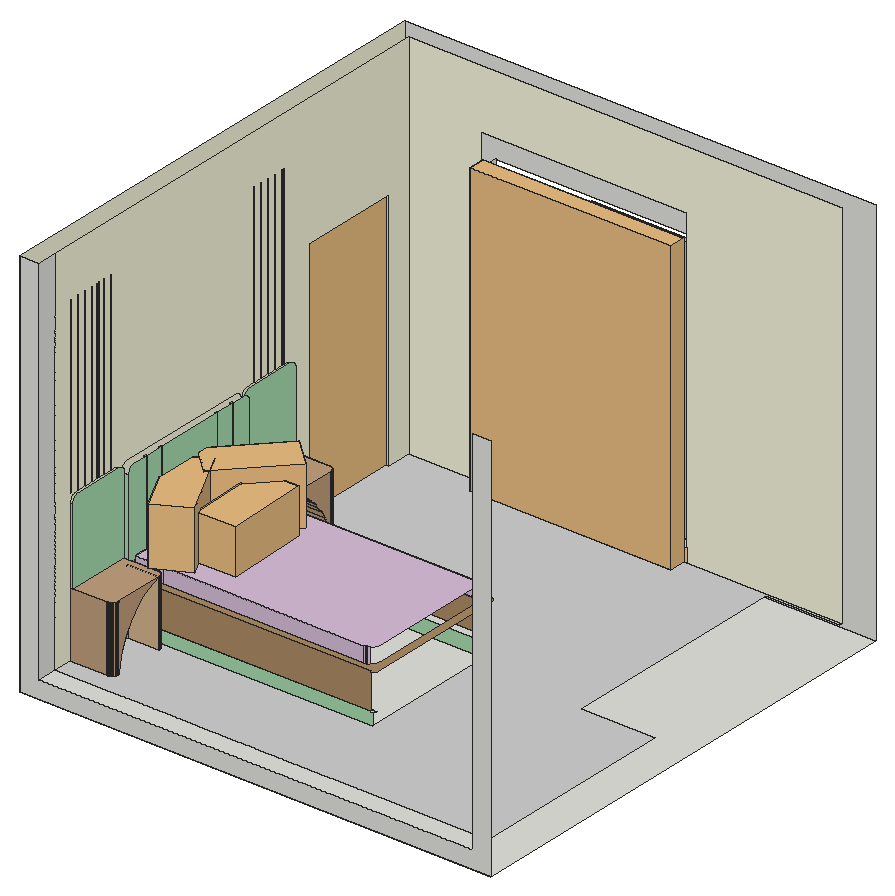
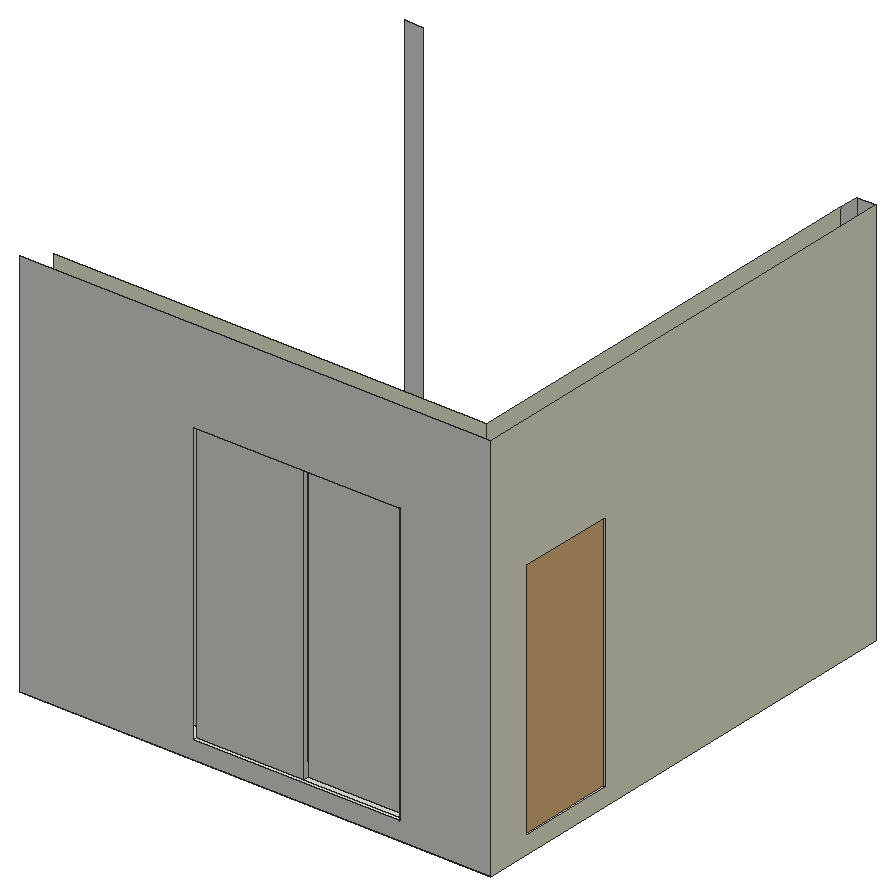
# SketchUp Ruby script. Lengths in inches.
U = 1.inch
M = Sketchup.active_model
def pt(a) = Geom::Point3d.new(a.map { |v| v * U })
def face(e, loops, mat)
  f = e.add_face(loops[0].map { |a| pt(a) })
  loops[1..].each { |l| e.add_face(l.map { |a| pt(a) }).erase! }
  f.material = f.back_material = mat if mat
  f
end
# faces: each face lists its corners as indices into pts; further lists are holes
def faces(e, pts, list, mat = nil) = list.each { |f| face(e, (f[0].is_a?(Array) ? f : [f]).map { |l| l.map { |i| pts[i] } }, mat) }
# xy, xz, yz: faces in a plane at the given z, y or x. An outline is a flat list of corners, or four numbers for a rectangle; further outlines are holes
def ring(l) = l.size == 4 ? [[l[0], l[1]], [l[2], l[1]], [l[2], l[3]], [l[0], l[3]]] : l.each_slice(2).to_a
def flat(e, list, mat, &to3) = list.each { |f| face(e, (f[0].is_a?(Array) ? f : [f]).map { |l| ring(l).map { |u, v| to3.(u, v) } }, mat) }
def xy(e, z, list, mat = nil) = flat(e, list, mat) { |x, y| [x, y, z] }
def xz(e, y, list, mat = nil) = flat(e, list, mat) { |x, z| [x, y, z] }
def yz(e, x, list, mat = nil) = flat(e, list, mat) { |y, z| [x, y, z] }
def lines(e, pts, list) = list.each { |a, b| e.add_line(pt(pts[a]), pt(pts[b])) }
# prism: a flat outline (further loops are holes) pulled along v
def prism(e, loops, v, mat = nil)
  f = face(e, loops, mat); d = Geom::Vector3d.new(v.map { |x| x * U })
  f.pushpull(f.normal.samedirection?(d) ? d.length : -d.length)
end
def box(e, o, s, mat = nil) = prism(e, [[o, [o[0] + s[0], o[1], o[2]], [o[0] + s[0], o[1] + s[1], o[2]], [o[0], o[1] + s[1], o[2]]]], [0, 0, s[2]], mat)
def at(x, y, z, deg = 0) = Geom::Transformation.translation(pt([x, y, z])) * Geom::Transformation.rotation(ORIGIN, Z_AXIS, deg.degrees)
def axes(o, x, y, z) = Geom::Transformation.new([*x, 0, *y, 0, *z, 0, *pt(o).to_a, 1])
def part(name) = M.definitions.add(name)
# library, detail: a bought-in or finely detailed component or shape, given as its bounding box
def library(name, o, s) = part(name).tap { |d| box(d.entities, o, s) }
def detail(e, o, s) = box(e.add_group.entities, o, s)
def put(e, d, t, mat = nil) = e.add_instance(d, t).tap { |i| i.material = mat if mat }
def group(e, t, mat = nil) = e.add_group.tap { |g| g.transformation = t; g.material = mat if mat }.entities
root = M.entities
M.materials.add("Glass Tinted Orange").color = [0, 0, 0]
M.materials["Glass Tinted Orange"].alpha = 0.13
M.materials.add("Leather K01 Brown 12cm").color = [167, 219, 175]
M.materials.add("Maquette Wood B01 12cm\#2").color = [172, 139, 100]
M.materials.add("Plywood B 50cm").color = [193, 159, 125]
M.materials.add("[0035_Tan]").color = [210, 180, 140]
M.materials.add("[0049_Beige]").color = [245, 245, 220]
M.materials.add("[0118_Thistle]").color = [216, 191, 216]
M.materials.add("[Carrera Marble]").color = [207, 207, 207]
M.materials.add("[Color C02]").color = [255, 204, 153]
c1 = library("door+(2)",[23.55,-155.59,32.04],[5.91,42.06,102.36])
c2 = library("Pillows 001",[-21.03,-6.66,0],[42.06,13.32,14.16])
c3 = library("Pillow 004",[-13.24,-4.32,0.02],[26.5,8.4,10.71])
c4 = library("Curtains",[207.47,199.36,7.375],[85.87,10.88,122.26])
xy(root,0,[[0,2.25,198.9375,205.19]])
xy(root,7.375,[[8.12,2.25,191.13,10.37],[23.49,105.14,26.49,105.14,26.49,112.01,26.47,111.62,26.39,111.23,26.26,110.86,26.09,110.51,25.87,110.18,25.61,109.89,25.32,109.63,24.99,109.41,24.64,109.24,24.27,109.11,23.88,109.04,23.49,109.01],[26.49,133.01,26.49,136.01,23.49,136.01,23.88,135.99,24.27,135.91,24.64,135.78,24.99,135.61,25.32,135.39,25.61,135.13,25.87,134.84,26.09,134.51,26.26,134.16,26.39,133.79,26.47,133.4],[38.58,200.94,80.73,203.13],[38.58,203.13,125.77,205.19]])
xy(root,7.375,[[8.12,10.37,191.13,10.37,191.13,98.61,159.88,98.61,159.88,195.82,191.32,195.82,191.32,197.07,8.12,197.07,8.12,186.76,0,186.76,0,144.7,8.12,144.7,8.12,136.01,26.49,136.01,26.49,133.01,15.12,133.01,15.12,112.01,26.49,112.01,26.49,105.14,113.43,105.14,113.43,46.51,23.49,46.51,23.49,45.51,23.88,45.49,24.27,45.41,24.64,45.28,24.99,45.11,25.32,44.89,25.61,44.63,25.87,44.34,26.09,44.01,26.26,43.66,26.39,43.29,26.47,42.9,26.49,42.51,13.24,42.51,13.24,21.51,26.49,21.51,26.47,21.12,26.39,20.73,26.26,20.36,26.09,20.01,25.87,19.68,25.61,19.39,25.32,19.13,24.99,18.91,24.64,18.74,24.27,18.61,23.88,18.54,23.49,18.51,8.12,18.51]],"[Carrera Marble]")
xy(root,13.0625,[[38.58,197.07,125.77,197.07,125.77,200.94,80.73,200.94,80.73,199,38.58,199]],"[Color C02]")
xy(root,13.375,[[23.49,45.51,23.68,46.51],[23.68,45.51,24.62,46.51],[24.62,45.51,24.62,46.51,115.06,46.51,115.05,46.48,114.9,46.27,114.74,46.08,114.55,45.91,114.34,45.77,114.11,45.66,113.87,45.58,113.62,45.53,113.37,45.51],[23.49,105.14,23.49,109.01,113.31,109.01,113.43,109,113.43,105.14]])
xy(root,28.5,[[10.74,54.26,11.43,55.26],[10.74,62.26,11.43,63.26],[10.74,91.64,11.43,92.64],[10.74,99.64,11.43,100.64]])
xy(root,28.5,[[11.43,45.51,113.37,45.51,113.62,45.53,113.87,45.58,114.11,45.66,114.34,45.77,114.55,45.91,114.74,46.08,114.9,46.27,115.05,46.48,115.16,46.71,115.24,46.95,115.29,47.2,115.31,47.45,115.31,107.01,115.29,107.27,115.24,107.53,115.15,107.78,115.04,108.01,114.89,108.23,114.72,108.43,114.52,108.6,114.31,108.74,114.07,108.86,113.82,108.94,113.57,108.99,113.31,109.01,11.43,109.01,11.43,105.76,108.06,105.76,108.58,105.73,109.09,105.625,109.59,105.46,110.06,105.22,110.49,104.93,110.88,104.59,111.23,104.2,111.52,103.76,111.75,103.29,111.92,102.8,112.02,102.28,112.06,101.76,112.06,52.76,112.02,52.24,111.92,51.73,111.75,51.23,111.52,50.76,111.23,50.33,110.88,49.93,110.49,49.59,110.06,49.3,109.59,49.07,109.09,48.9,108.58,48.8,108.06,48.76,11.43,48.76]],"Maquette Wood B01 12cm\#2")
xy(root,35,[[9.43,18.51,23.49,18.51,23.88,18.54,24.27,18.61,24.64,18.74,24.99,18.91,25.32,19.13,25.61,19.39,25.87,19.68,26.09,20.01,26.26,20.36,26.39,20.73,26.47,21.12,26.49,21.51,26.49,42.51,26.47,42.9,26.39,43.29,26.26,43.66,26.09,44.01,25.87,44.34,25.61,44.63,25.32,44.89,24.99,45.11,24.64,45.28,24.27,45.41,23.88,45.49,23.49,45.51,9.43,45.51],[9.43,109.01,23.49,109.01,23.88,109.04,24.27,109.11,24.64,109.24,24.99,109.41,25.32,109.63,25.61,109.89,25.87,110.18,26.09,110.51,26.26,110.86,26.39,111.23,26.47,111.62,26.49,112.01,26.49,133.01,26.47,133.4,26.39,133.79,26.26,134.16,26.09,134.51,25.87,134.84,25.61,135.13,25.32,135.39,24.99,135.61,24.64,135.78,24.27,135.91,23.88,135.99,23.49,136.01,9.43,136.01]],"Plywood B 50cm")
xy(root,35,[[11.43,48.76,108.06,48.76,108.58,48.8,109.09,48.9,109.59,49.07,110.06,49.3,110.49,49.59,110.88,49.93,111.23,50.33,111.52,50.76,111.75,51.23,111.92,51.73,112.02,52.24,112.06,52.76,112.06,101.76,112.02,102.28,111.92,102.8,111.75,103.29,111.52,103.76,111.23,104.2,110.88,104.59,110.49,104.93,110.06,105.22,109.59,105.46,109.09,105.625,108.58,105.73,108.06,105.76,11.43,105.76]],"[0118_Thistle]")
xz(root,2.25,[[0,0,198.9375,0,198.9375,164.75,191.13,164.75,191.13,7.375,8.12,7.375,8.12,164.75,0,164.75]])
xz(root,18.51,[[8.12,35,9.43,67.0625]],"Leather K01 Brown 12cm")
xz(root,18.51,[[8.12,7.375,23.49,35]],"Plywood B 50cm")
xz(root,42.51,[[13.24,7.375,26.49,35]],"[0035_Tan]")
xz(root,45.51,[[9.43,35,11.43,67.0625]],"Leather K01 Brown 12cm")
xz(root,45.51,[[23.49,13.375,113.37,28.5]],"Maquette Wood B01 12cm\#2")
xz(root,45.51,[[11.43,28.5,23.49,35]],"Plywood B 50cm")
xz(root,46.51,[[23.49,7.375,113.43,13.375]],"Leather K01 Brown 12cm")
xz(root,48.76,[[11.43,28.5,23.49,35],[23.49,28.5,108.06,35]],"[0118_Thistle]")
xz(root,54.26,[[10.74,28.5,11.43,70.0625]],"Leather K01 Brown 12cm")
xz(root,55.26,[[10.74,28.5,11.43,70.0625]],"Leather K01 Brown 12cm")
xz(root,62.26,[[10.74,28.5,11.43,70.0625]],"Leather K01 Brown 12cm")
xz(root,63.26,[[10.74,28.5,11.43,70.0625]],"Leather K01 Brown 12cm")
xz(root,91.64,[[10.74,28.5,11.43,70.0625]],"Leather K01 Brown 12cm")
xz(root,92.64,[[10.74,28.5,11.43,70.0625]],"Leather K01 Brown 12cm")
xz(root,99.64,[[10.74,28.5,11.43,70.0625]],"Leather K01 Brown 12cm")
xz(root,100.64,[[10.74,28.5,11.43,70.0625]],"Leather K01 Brown 12cm")
xz(root,105.14,[[23.49,7.375,113.43,13.375]],"Leather K01 Brown 12cm")
xz(root,105.76,[[11.43,28.5,23.49,35],[23.49,28.5,108.06,35]],"[0118_Thistle]")
xz(root,109.01,[[9.43,35,11.43,67.0625]],"Leather K01 Brown 12cm")
xz(root,109.01,[[23.49,13.375,113.31,28.5]],"Maquette Wood B01 12cm\#2")
xz(root,109.01,[[11.43,28.5,23.49,35]],"Plywood B 50cm")
xz(root,112.01,[[15.12,7.375,26.49,35]],"[0035_Tan]")
xz(root,136.01,[[8.12,35,9.43,67.0625]],"Leather K01 Brown 12cm")
xz(root,136.01,[[8.12,7.375,23.49,35]],"Plywood B 50cm")
xz(root,144.7,[[0,7.375,8.12,109.5625]])
xz(root,186.76,[[0,7.375,8.12,109.5625]])
xz(root,197.07,[[8.12,7.375,38.58,7.375,38.58,139.75,125.77,139.75,125.77,7.375,191.32,7.375,191.32,164.75,8.12,164.75]],"[0049_Beige]")
xz(root,197.07,[[38.58,7.375,125.77,13.0625]],"[Color C02]")
xz(root,199,[[38.58,13.0625,80.73,13.0625,80.73,126.5625,41.29,126.5625,41.29,125.75,38.58,125.75]],"Glass Tinted Orange")
xz(root,200.94,[[38.58,7.375,38.58,125.75,41.29,125.75,41.29,126.5625,80.73,126.5625,80.73,7.375]])
xz(root,200.94,[[80.73,13.0625,125.77,125.75]],"Glass Tinted Orange")
xz(root,203.13,[[80.73,7.375,125.77,125.75]])
xz(root,205.19,[[[0,0,198.9375,164.75],[38.58,7.375,125.77,125.75]]])
yz(root,0,[[[2.25,0,205.19,164.75],[144.7,7.375,186.76,109.5625]]],"[0049_Beige]")
yz(root,8.12,[[2.25,7.375,10.37,164.75]])
yz(root,8.12,[[[10.37,7.375,18.51,7.375,18.51,67.0625,18.54,67.45,18.61,67.84,18.74,68.21,18.91,68.5625,19.13,68.89,19.39,69.18,19.68,69.44,20.01,69.66,20.36,69.83,20.73,69.96,21.12,70.04,21.51,70.0625,22.24,70.0625,22.24,144.0625,23.01,144.0625,23.01,70.0625,23.49,70.0625,23.49,144.0625,24.25,144.0625,24.25,70.0625,24.73,70.0625,24.73,144.0625,25.5,144.0625,25.5,70.0625,25.98,70.0625,25.98,144.0625,26.74,144.0625,26.74,70.0625,27.22,70.0625,27.22,144.0625,27.99,144.0625,27.99,70.0625,28.47,70.0625,28.47,144.0625,29.23,144.0625,29.23,70.0625,29.71,70.0625,29.71,144.0625,30.48,144.0625,30.48,70.0625,30.95,70.0625,30.95,144.0625,31.72,144.0625,31.72,70.0625,32.2,70.0625,32.2,144.0625,32.97,144.0625,32.97,70.0625,33.44,70.0625,33.44,144.0625,34.21,144.0625,34.21,70.0625,34.6875,70.0625,34.6875,144.0625,35.45,144.0625,35.45,70.0625,35.93,70.0625,35.93,144.0625,36.7,144.0625,36.7,70.0625,37.18,70.0625,37.18,144.0625,37.94,144.0625,37.94,70.0625,38.42,70.0625,38.42,144.0625,39.1875,144.0625,39.1875,70.0625,39.66,70.0625,39.66,144.0625,40.43,144.0625,40.43,70.0625,40.91,70.0625,40.91,144.0625,41.68,144.0625,41.68,70.0625,42.51,70.0625,42.9,70.04,43.29,69.96,43.66,69.83,44.01,69.66,44.34,69.44,44.63,69.18,44.89,68.89,45.11,68.5625,45.28,68.21,45.41,67.84,45.49,67.45,45.51,67.0625,45.54,67.45,45.61,67.84,45.74,68.21,45.91,68.5625,46.13,68.89,46.39,69.18,46.68,69.44,47.01,69.66,47.36,69.83,47.73,69.96,48.12,70.04,48.51,70.0625,106.01,70.0625,106.4,70.04,106.79,69.96,107.16,69.83,107.51,69.66,107.84,69.44,108.13,69.18,108.39,68.89,108.61,68.5625,108.78,68.21,108.91,67.84,108.99,67.45,109.01,67.0625,109.04,67.45,109.11,67.84,109.24,68.21,109.41,68.5625,109.63,68.89,109.89,69.18,110.18,69.44,110.51,69.66,110.86,69.83,111.23,69.96,111.62,70.04,112.01,70.0625,112.69,70.0625,112.69,144.0625,113.46,144.0625,113.46,70.0625,113.92,70.0625,113.92,144.0625,114.6875,144.0625,114.6875,70.0625,115.15,70.0625,115.15,144.0625,115.91,144.0625,115.91,70.0625,116.375,70.0625,116.375,144.0625,117.14,144.0625,117.14,70.0625,117.6,70.0625,117.6,144.0625,118.37,144.0625,118.37,70.0625,118.83,70.0625,118.83,144.0625,119.6,144.0625,119.6,70.0625,120.06,70.0625,120.06,144.0625,120.82,144.0625,120.82,70.0625,121.28,70.0625,121.28,144.0625,122.05,144.0625,122.05,70.0625,122.51,70.0625,122.51,144.0625,123.28,144.0625,123.28,70.0625,123.74,70.0625,123.74,144.0625,124.5,144.0625,124.5,70.0625,124.97,70.0625,124.97,144.0625,125.73,144.0625,125.73,70.0625,126.19,70.0625,126.19,144.0625,126.96,144.0625,126.96,70.0625,127.42,70.0625,127.42,144.0625,128.1875,144.0625,128.1875,70.0625,128.65,70.0625,128.65,144.0625,129.41,144.0625,129.41,70.0625,129.875,70.0625,129.875,144.0625,130.64,144.0625,130.64,70.0625,131.1,70.0625,131.1,144.0625,131.87,144.0625,131.87,70.0625,133.01,70.0625,133.4,70.04,133.79,69.96,134.16,69.83,134.51,69.66,134.84,69.44,135.13,69.18,135.39,68.89,135.61,68.5625,135.78,68.21,135.91,67.84,135.99,67.45,136.01,67.0625,136.01,7.375,144.7,7.375,144.7,109.5625,186.76,109.5625,186.76,7.375,197.07,7.375,197.07,164.75,10.37,164.75],[18.51,70.0625,19.28,144.0625]]],"[0049_Beige]")
yz(root,9.43,[[18.51,35,45.51,35,45.51,67.0625,45.49,67.45,45.41,67.84,45.28,68.21,45.11,68.5625,44.89,68.89,44.63,69.18,44.34,69.44,44.01,69.66,43.66,69.83,43.29,69.96,42.9,70.04,42.51,70.0625,21.51,70.0625,21.12,70.04,20.73,69.96,20.36,69.83,20.01,69.66,19.68,69.44,19.39,69.18,19.13,68.89,18.91,68.5625,18.74,68.21,18.61,67.84,18.54,67.45,18.51,67.0625],[109.01,35,136.01,35,136.01,67.0625,135.99,67.45,135.91,67.84,135.78,68.21,135.61,68.5625,135.39,68.89,135.13,69.18,134.84,69.44,134.51,69.66,134.16,69.83,133.79,69.96,133.4,70.04,133.01,70.0625,112.01,70.0625,111.62,70.04,111.23,69.96,110.86,69.83,110.51,69.66,110.18,69.44,109.89,69.18,109.63,68.89,109.41,68.5625,109.24,68.21,109.11,67.84,109.04,67.45,109.01,67.0625]],"Leather K01 Brown 12cm")
yz(root,10.74,[[54.26,28.5,55.26,70.0625],[62.26,28.5,63.26,70.0625],[91.64,28.5,92.64,70.0625],[99.64,28.5,100.64,70.0625]],"Leather K01 Brown 12cm")
yz(root,11.43,[[48.76,28.5,54.26,35],[54.26,28.5,55.26,35],[55.26,28.5,57.51,35],[57.51,28.5,62.26,35],[62.26,28.5,63.26,35],
  [63.26,28.5,65.51,35],[65.51,28.5,91.64,35],[91.64,28.5,92.64,35],[92.64,28.5,94.89,35],[94.89,28.5,99.64,35],
  [99.64,28.5,100.64,35],[100.64,28.5,102.89,35]])
yz(root,11.43,[[45.51,28.5,48.76,28.5,48.76,35,54.26,35,54.26,70.0625,48.51,70.0625,48.12,70.04,47.73,69.96,47.36,69.83,47.01,69.66,46.68,69.44,46.39,69.18,46.13,68.89,45.91,68.5625,45.74,68.21,45.61,67.84,45.54,67.45,45.51,67.0625],[105.76,28.5,109.01,28.5,109.01,67.0625,108.99,67.45,108.91,67.84,108.78,68.21,108.61,68.5625,108.39,68.89,108.13,69.18,107.84,69.44,107.51,69.66,107.16,69.83,106.79,69.96,106.4,70.04,106.01,70.0625,100.64,70.0625,100.64,35,105.76,35],[55.26,35,62.26,70.0625],[63.26,35,91.64,70.0625],[92.64,35,99.64,70.0625]],"Leather K01 Brown 12cm")
yz(root,13.24,[[21.51,7.375,42.51,7.375,42.51,35,39.62,33.93,36.85,32.57,34.24,30.93,31.81,29.04,29.59,26.9,27.6,24.54,25.86,22,24.39,19.28,23.22,16.43,22.34,13.48,21.77,10.45]],"[0035_Tan]")
yz(root,15.12,[[112.01,7.375,133.01,7.375,132.63,10.41,131.97,13.39,131.02,16.3,129.8,19.1,128.32,21.77,126.59,24.29,124.63,26.63,122.45,28.77,120.08,30.7,117.53,32.39,114.83,33.83,112.01,35]],"[0035_Tan]")
yz(root,23.49,[[45.51,7.375,46.51,13.375],[105.14,7.375,109.01,13.375]],"Leather K01 Brown 12cm")
yz(root,26.49,[[21.51,7.375,21.77,10.45,22.34,13.48,23.22,16.43,24.39,19.28,25.86,22,27.6,24.54,29.59,26.9,31.81,29.04,34.24,30.93,36.85,32.57,39.62,33.93,42.51,35,21.51,35],[133.01,7.375,133.01,35,112.01,35,114.83,33.83,117.53,32.39,120.08,30.7,122.45,28.77,124.63,26.63,126.59,24.29,128.32,21.77,129.8,19.1,131.02,16.3,131.97,13.39,132.63,10.41]],"Plywood B 50cm")
yz(root,38.58,[[200.94,7.375,205.19,125.75],[197.07,13.0625,199,125.75]])
yz(root,80.73,[[200.94,7.375,203.13,125.75]])
yz(root,80.73,[[199,13.0625,200.94,126.5625]],"Glass Tinted Orange")
p = [[23.88,18.54,35],[23.49,18.51,35],[23.49,18.51,7.375],[23.88,18.54,7.375],[24.27,18.61,35],[24.27,18.61,7.375],
  [24.64,18.74,35],[24.64,18.74,7.375],[24.99,18.91,35],[24.99,18.91,7.375],[25.32,19.13,35],[25.32,19.13,7.375],
  [25.61,19.39,35],[25.61,19.39,7.375],[25.87,19.68,35],[25.87,19.68,7.375],[26.09,20.01,35],[26.09,20.01,7.375],
  [26.26,20.36,35],[26.26,20.36,7.375],[26.39,20.73,35],[26.39,20.73,7.375],[26.47,21.12,35],[26.47,21.12,7.375],
  [26.49,21.51,35],[26.49,21.51,7.375],[26.49,21.77,10.45],[13.24,21.51,7.375],[13.24,21.77,10.45],[26.47,42.9,35],
  [26.49,42.51,35],[26.49,42.51,7.375],[26.47,42.9,7.375],[26.39,43.29,35],[26.39,43.29,7.375],[26.26,43.66,35],
  [26.26,43.66,7.375],[26.09,44.01,35],[26.09,44.01,7.375],[25.87,44.34,35],[25.87,44.34,7.375],[25.61,44.63,35],
  [25.61,44.63,7.375],[25.32,44.89,35],[25.32,44.89,7.375],[24.99,45.11,35],[24.99,45.11,7.375],[24.64,45.28,35],
  [24.64,45.28,7.375],[24.27,45.41,35],[24.27,45.41,7.375],[23.88,45.49,35],[23.88,45.49,7.375],[23.49,45.51,35],
  [23.49,45.51,7.375],[23.49,45.51,13.375],[23.49,45.51,28.5],[23.88,109.04,35],[23.49,109.01,35],[23.49,109.01,28.5],
  [23.49,109.01,13.375],[23.49,109.01,7.375],[23.88,109.04,7.375],[24.27,109.11,35],[24.27,109.11,7.375],[24.64,109.24,35],
  [24.64,109.24,7.375],[24.99,109.41,35],[24.99,109.41,7.375],[25.32,109.63,35],[25.32,109.63,7.375],[25.61,109.89,35],
  [25.61,109.89,7.375],[25.87,110.18,35],[25.87,110.18,7.375],[26.09,110.51,35],[26.09,110.51,7.375],[26.26,110.86,35],
  [26.26,110.86,7.375],[26.39,111.23,35],[26.39,111.23,7.375],[26.47,111.62,35],[26.47,111.62,7.375],[26.49,112.01,35],
  [26.49,112.01,7.375],[26.49,133.01,7.375],[26.49,132.63,10.41],[15.12,132.63,10.41],[15.12,133.01,7.375],[26.47,133.4,35],
  [26.49,133.01,35],[26.47,133.4,7.375],[26.39,133.79,35],[26.39,133.79,7.375],[26.26,134.16,35],[26.26,134.16,7.375],
  [26.09,134.51,35],[26.09,134.51,7.375],[25.87,134.84,35],[25.87,134.84,7.375],[25.61,135.13,35],[25.61,135.13,7.375],
  [25.32,135.39,35],[25.32,135.39,7.375],[24.99,135.61,35],[24.99,135.61,7.375],[24.64,135.78,35],[24.64,135.78,7.375],
  [24.27,135.91,35],[24.27,135.91,7.375],[23.88,135.99,35],[23.88,135.99,7.375],[23.49,136.01,35],[23.49,136.01,7.375],
  [26.49,22.34,13.48],[13.24,22.34,13.48],[26.49,131.97,13.39],[15.12,131.97,13.39],[26.49,131.02,16.3],[15.12,131.02,16.3],
  [26.49,23.22,16.43],[13.24,23.22,16.43],[26.49,129.8,19.1],[15.12,129.8,19.1],[26.49,24.39,19.28],[13.24,24.39,19.28],
  [26.49,128.32,21.77],[15.12,128.32,21.77],[26.49,25.86,22],[13.24,25.86,22],[26.49,126.59,24.29],[15.12,126.59,24.29],
  [26.49,27.6,24.54],[13.24,27.6,24.54],[26.49,124.63,26.63],[15.12,124.63,26.63],[26.49,29.59,26.9],[13.24,29.59,26.9],
  [26.49,122.45,28.77],[15.12,122.45,28.77],[26.49,31.81,29.04],[13.24,31.81,29.04],[108.58,48.8,35],[108.06,48.76,35],
  [108.06,48.76,28.5],[108.58,48.8,28.5],[109.09,48.9,35],[109.09,48.9,28.5],[109.59,49.07,35],[109.59,49.07,28.5],
  [110.06,49.3,35],[110.06,49.3,28.5],[109.59,105.46,35],[110.06,105.22,35],[110.06,105.22,28.5],[109.59,105.46,28.5],
  [109.09,105.625,35],[109.09,105.625,28.5],[108.58,105.73,35],[108.58,105.73,28.5],[108.06,105.76,35],[108.06,105.76,28.5],
  [26.49,120.08,30.7],[15.12,120.08,30.7],[26.49,34.24,30.93],[13.24,34.24,30.93],[26.49,117.53,32.39],[15.12,117.53,32.39],
  [26.49,36.85,32.57],[13.24,36.85,32.57],[26.49,114.83,33.83],[15.12,114.83,33.83],[26.49,39.62,33.93],[13.24,39.62,33.93],
  [15.12,112.01,35],[13.24,42.51,35]]
faces(root,p,[[0,1,2,3],[4,0,3,5],[6,4,5,7],[8,6,7,9],[10,8,9,11],[12,10,11,13],[14,12,13,15],[16,14,15,17],
  [18,16,17,19],[20,18,19,21],[22,20,21,23],[24,22,23,25],[29,30,31,32],[33,29,32,34],[35,33,34,36],[37,35,36,38],
  [39,37,38,40],[41,39,40,42],[43,41,42,44],[45,43,44,46],[47,45,46,48],[49,47,48,50],[51,49,50,52],[53,51,52,54,55,56],
  [57,58,59,60,61,62],[63,57,62,64],[65,63,64,66],[67,65,66,68],[69,67,68,70],[71,69,70,72],[73,71,72,74],[75,73,74,76],
  [77,75,76,78],[79,77,78,80],[81,79,80,82],[83,81,82,84],[89,90,85,91],[92,89,91,93],[94,92,93,95],[96,94,95,97],
  [98,96,97,99],[100,98,99,101],[102,100,101,103],[104,102,103,105],[106,104,105,107],[108,106,107,109],[110,108,109,111],[112,110,111,113]],"Plywood B 50cm")
faces(root,p,[[26,25,27,28],[85,86,87,88],[114,26,28,115],[86,116,117,87],[116,118,119,117],[120,114,115,121],[118,122,123,119],[124,120,121,125],
  [122,126,127,123],[128,124,125,129],[126,130,131,127],[132,128,129,133],[130,134,135,131],[136,132,133,137],[134,138,139,135],[140,136,137,141],
  [138,162,163,139],[164,140,141,165],[162,166,167,163],[168,164,165,169],[166,170,171,167],[172,168,169,173],[170,83,174,171],[30,172,173,175]],"[0035_Tan]")
faces(root,p,[[142,143,144,145],[146,142,145,147],[148,146,147,149],[150,148,149,151]],"[0118_Thistle]")
faces(root,p,[[152,153,154,155],[156,152,155,157],[158,156,157,159],[160,158,159,161]])
put(root,c1,at(-22.45,300.29,-24.84))
put(root,c2,axes([19.06,63.65,35],[-0.36829,0.71661,0],[-1.03857,-0.53375,0],[0,0,1.71704]))
put(root,c2,axes([26.55,91.06,35.28],[0.54959,0.58917,0],[-0.85387,0.79651,0],[0,0,1.71704]))
put(root,c3,axes([37.22,75.48,34.97],[-0.0362,1.3076,0],[-1.9614,-0.0543,0],[0,0,1.75181]))
put(root,c4,axes([-165.04,62.52,0],[0.98684,0,0],[0,0.64,0],[0,0,1]))
